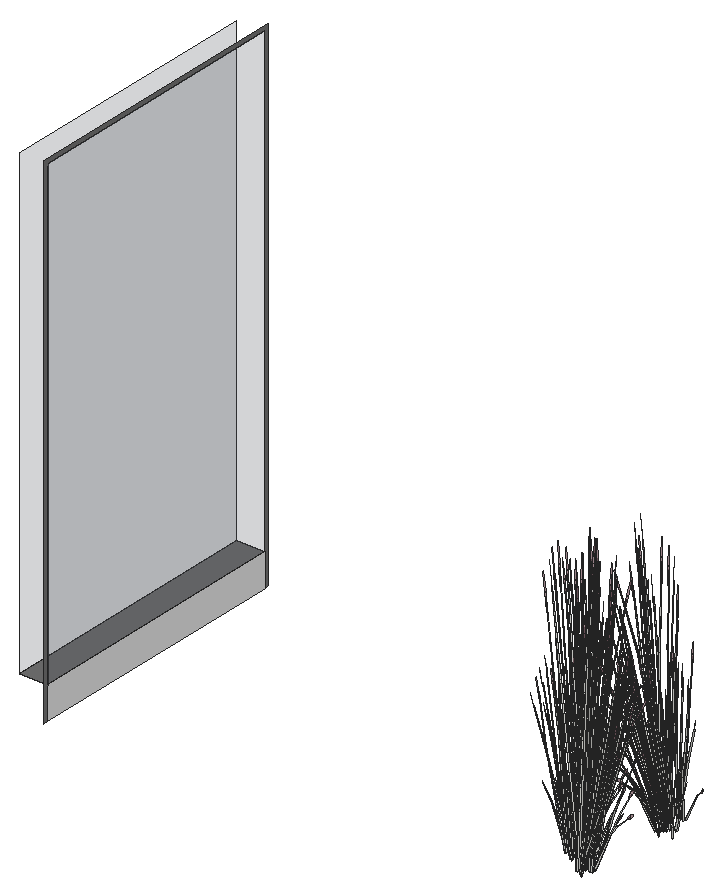
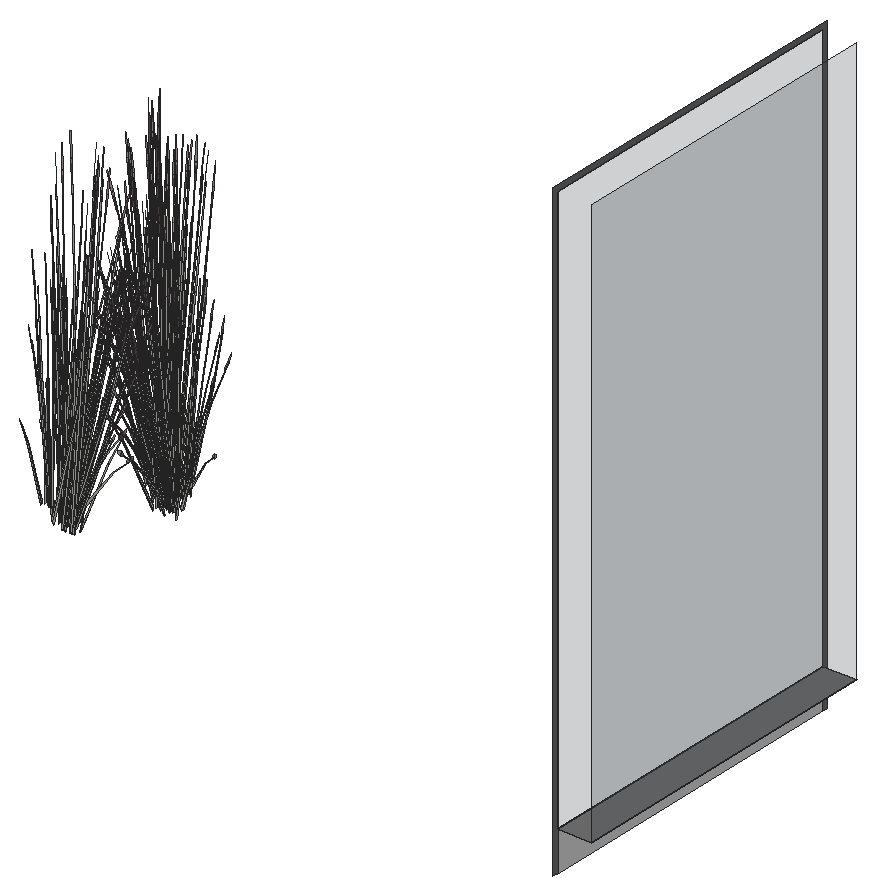
# SketchUp Ruby script. Lengths in inches.
U = 1.inch
M = Sketchup.active_model
def pt(a) = Geom::Point3d.new(a.map { |v| v * U })
def face(e, loops, mat)
  f = e.add_face(loops[0].map { |a| pt(a) })
  loops[1..].each { |l| e.add_face(l.map { |a| pt(a) }).erase! }
  f.material = f.back_material = mat if mat
  f
end
# faces: each face lists its corners as indices into pts; further lists are holes
def faces(e, pts, list, mat = nil) = list.each { |f| face(e, (f[0].is_a?(Array) ? f : [f]).map { |l| l.map { |i| pts[i] } }, mat) }
# xy, xz, yz: faces in a plane at the given z, y or x. An outline is a flat list of corners, or four numbers for a rectangle; further outlines are holes
def ring(l) = l.size == 4 ? [[l[0], l[1]], [l[2], l[1]], [l[2], l[3]], [l[0], l[3]]] : l.each_slice(2).to_a
def flat(e, list, mat, &to3) = list.each { |f| face(e, (f[0].is_a?(Array) ? f : [f]).map { |l| ring(l).map { |u, v| to3.(u, v) } }, mat) }
def xy(e, z, list, mat = nil) = flat(e, list, mat) { |x, y| [x, y, z] }
def xz(e, y, list, mat = nil) = flat(e, list, mat) { |x, z| [x, y, z] }
def yz(e, x, list, mat = nil) = flat(e, list, mat) { |y, z| [x, y, z] }
def lines(e, pts, list) = list.each { |a, b| e.add_line(pt(pts[a]), pt(pts[b])) }
# prism: a flat outline (further loops are holes) pulled along v
def prism(e, loops, v, mat = nil)
  f = face(e, loops, mat); d = Geom::Vector3d.new(v.map { |x| x * U })
  f.pushpull(f.normal.samedirection?(d) ? d.length : -d.length)
end
def box(e, o, s, mat = nil) = prism(e, [[o, [o[0] + s[0], o[1], o[2]], [o[0] + s[0], o[1] + s[1], o[2]], [o[0], o[1] + s[1], o[2]]]], [0, 0, s[2]], mat)
def at(x, y, z, deg = 0) = Geom::Transformation.translation(pt([x, y, z])) * Geom::Transformation.rotation(ORIGIN, Z_AXIS, deg.degrees)
def axes(o, x, y, z) = Geom::Transformation.new([*x, 0, *y, 0, *z, 0, *pt(o).to_a, 1])
def part(name) = M.definitions.add(name)
# library, detail: a bought-in or finely detailed component or shape, given as its bounding box
def library(name, o, s) = part(name).tap { |d| box(d.entities, o, s) }
def detail(e, o, s) = box(e.add_group.entities, o, s)
def put(e, d, t, mat = nil) = e.add_instance(d, t).tap { |i| i.material = mat if mat }
def group(e, t, mat = nil) = e.add_group.tap { |g| g.transformation = t; g.material = mat if mat }.entities
root = M.entities
M.materials.add("Glass_Basic_01").color = [105, 113, 122]
M.materials["Glass_Basic_01"].alpha = 0.25
M.materials.add("LightPink_Translucent").color = [144, 107, 117]
M.materials["LightPink_Translucent"].alpha = 0.75
M.materials.add("M01_Silver_Fog").color = [224, 224, 224]
M.materials.add("M06_Steel_Smoke").color = [114, 114, 114]
c1 = part("blade")
p = [[2.15,0.21,22],[0,0.17,0],[0.09,0.45,0],[2.18,0.31,22],[2.29,0.31,22],[0.38,0.45,0],
  [2.48,0.24,33],[2.49,0.24,33],[2.48,0.22,33]]
faces(c1.entities,p,[[0,1,2,3],[4,5,2,3],[6,3,4,7],[8,0,3,6]])
c2 = part("seeds")
p = [[0.3,-0.1,1.38],[-0.01,-0.03,1.59],[-0.01,-0.03,0.03],[0.14,-0.07,-0.07],[0.29,-0.03,3],[0.15,0.01,3.11]]
faces(c2.entities,p,[[0,1,2,3],[1,0,4,5]],"LightPink_Translucent")
c3 = part("blade with seeds")
put(c3.entities,c1,at(0,0,0))
put(c3.entities,c2,axes([2.4,0.25,30.99],[1.5799,-0.05474,1.17369],[-0.12525,1.92788,0.29478],[-0.07173,-0.02425,1.56792]))
xy(root,277,[[204,295,210,353]],"M06_Steel_Smoke")
yz(root,204,[[295,277,353,377]],"Glass_Basic_01")
yz(root,210,[[295,277,353,377]],"Glass_Basic_01")
yz(root,210,[[295,270,353,277]],"M01_Silver_Fog")
yz(root,210,[[294,270,295,270,295,377,353,377,353,270,354,270,354,378,294,378]],"M06_Steel_Smoke")
put(root,c3,axes([315.625,308.53,274.53],[0.41757,0.15024,-0.35414],[-0.12179,0.4383,0.4572],[0.16812,-0.04019,0.87481]))
put(root,c3,axes([311.76,309.83,272.02],[-0.47024,-0.26927,-0.49651],[0.28107,-0.48284,0],[-0.1071,-0.06133,1.57504]))
put(root,c3,axes([314.89,306.64,272.02],[0.47024,0.26927,-0.49651],[-0.28107,0.48284,0],[0.1071,0.06133,1.57504]))
put(root,c3,axes([310.72,307.83,274.53],[-0.41757,-0.15024,-0.35414],[0.12179,-0.4383,0.4572],[-0.16812,0.04019,0.87481]))
put(root,c3,axes([313.99,308.17,272.21],[0.56215,0,0],[0,0.55754,0],[0,0,1.78407]))
put(root,c3,axes([313.04,308.875,272.67],[-0.5073,0.35754,-0.29095],[-0.33735,-0.5052,-0.50002],[-0.12516,-0.05131,1.59708]))
put(root,c3,axes([314.15,306.87,272.47],[-0.53992,0.14294,0.17642],[-0.13332,-0.53195,0.35086],[0.04815,0.07751,1.60407]))
put(root,c3,axes([314.49,307.99,273.875],[-0.20841,0.0122,1.71376],[0.13825,-0.52864,0.13857],[0.297,0.0327,0.73262]))
put(root,c3,axes([314.75,306.84,272.03],[0.11803,0.46926,-0.30978],[-0.46876,0.13325,0.30978],[0.0945,0.05411,1.38974]))
put(root,c3,axes([315.5625,308.71,274.73],[0.18454,0.3672,0.0643],[-0.33652,0.17973,0.50621],[0.14834,-0.03546,0.77189]))
put(root,c3,axes([313.8125,307.89,272.38],[-0.63506,-0.11347,0.49198],[0.12924,-0.64083,0.19306],[0.09281,0.06188,1.70813]))
put(root,c3,axes([315.53,308.58,274.73],[-0.14195,0.49104,0.48003],[-0.46669,-0.16791,0.3958],[0.18353,-0.02951,0.9933]))
put(root,c3,axes([313.3,309.47,272.2],[-0.16394,-0.4643,0],[0.46814,-0.1626,0],[0,0,1.54371]))
put(root,c3,axes([312.99,309.03,272.62],[-0.09693,0.48062,0.1448],[-0.47357,-0.08343,-0.41347],[-0.08619,-0.04935,1.26744]))
put(root,c3,axes([311.16,307.78,275.05],[0.41757,0.15024,0.35414],[-0.12179,0.4383,-0.4572],[-0.16812,0.04019,0.87481]))
put(root,c3,axes([313.92,309.41,272.18],[0.5275,-0.18273,-0.19198],[0.18536,0.52636,0.00008],[0.05823,-0.0202,1.73897]))
put(root,c3,axes([314.1,309.625,272.47],[0.14515,-0.53522,0.17642],[0.53115,0.15146,0.35086],[-0.09175,0.00261,1.60407]))
put(root,c3,axes([313.98,308.41,272.21],[0.35073,0.34786,0],[-0.35073,0.34786,0],[0,0,1.69266]))
put(root,c3,axes([311.99,307.76,273.34],[0.14282,-0.0779,1.77064],[0.04925,0.54394,0.13857],[-0.30935,0.07218,0.63284]))
put(root,c3,axes([314.93,308.26,272.47],[-0.39477,-0.39228,0.17642],[0.39783,-0.38049,0.35086],[-0.0436,0.08011,1.60407]))
put(root,c3,axes([314.2,307.67,272.06],[0.52267,0.08829,-0.62353],[-0.11029,0.54463,-0.16365],[0.15598,0.06599,1.37633]))
put(root,c3,axes([316.51,308.62,272.77],[-0.31044,0.08891,1.1486],[0.14613,-0.36744,0.84392],[0.16469,0.02514,0.25299]))
put(root,c3,axes([313.1875,309.68,272.2],[-0.50654,-0.24178,0],[0.24378,-0.50239,0],[0,0,1.62707]))
put(root,c3,axes([313.61,309.04,272.46],[-0.49063,-0.43346,-0.25192],[0.41285,-0.48673,0.5513],[-0.13212,0.05071,1.68216]))
put(root,c3,axes([312.32,309.87,272.48],[0.47024,0.26927,0.49651],[-0.28107,0.48284,0],[-0.1071,-0.06133,1.57504]))
put(root,c3,axes([313.98,308.01,272.72],[0.24378,-0.48527,0.44739],[0.50654,0.23354,-0.21531],[0,0.11186,1.43643]))
put(root,c3,axes([316.36,310.17,274.71],[-0.04543,-0.04715,1.77383],[0.09938,-0.50538,-0.16761],[0.17896,-0.03229,0.31391]))
put(root,c3,axes([310.45,308.125,274.72],[-0.08205,0.06992,1.74944],[0.00698,0.51086,-0.27667],[-0.18807,0.06644,0.14031]))
put(root,c3,axes([313.88,308.28,272.29],[0,0.62282,-0.05637],[-0.62828,0,0],[0,0.01957,1.79368]))
put(root,c3,axes([311,308.06,274.68],[-0.13612,0.48987,-0.51099],[-0.46669,-0.16791,-0.3958],[-0.1879,0.04492,0.97773]))
put(root,c3,axes([310.98,307.64,275.03],[0.25281,0.48765,-0.1216],[-0.44869,0.23964,-0.67495],[-0.18908,0.06434,1.02557]))
put(root,c3,axes([313.93,307.84,272.21],[0.30184,0.45202,-0.44739],[-0.45719,0.31831,0.21531],[0.09768,0.05593,1.43643]))
put(root,c3,axes([315.97,309.75,273.93],[-0.09617,-0.45271,-0.03492],[0.45453,-0.10408,-0.15832],[0.09492,0.0287,0.52218]))
put(root,c3,axes([312.05,310.15,272.375],[-0.31414,0.53965,0],[-0.52557,-0.30095,-0.51607],[-0.1197,-0.06854,1.63711]))
put(root,c3,axes([314.79,309.74,275.03],[0.0269,-0.54769,-0.1216],[0.50939,0.01497,-0.67495],[0.19618,0.03804,1.02557]))
put(root,c3,axes([315.26,308.28,272.48],[0,-0.53854,0.49651],[0.56215,0,0],[0,0.12266,1.57504]))
put(root,c3,axes([313.85,308.68,272.72],[0.54562,-0.03324,0.44739],[0.04934,0.55185,-0.21531],[-0.09768,0.05593,1.43643]))
put(root,c3,axes([314.1875,308.12,272.62],[0.46814,-0.15705,0.1448],[0.16394,0.44848,-0.41347],[0,0.0987,1.26744]))
put(root,c3,axes([314.71,309.52,275.05],[-0.28589,-0.33718,0.35414],[0.32644,-0.31919,-0.4572],[0.16586,0.04856,0.87481]))
put(root,c3,axes([313.36,308.95,272.21],[-0.54562,0.03324,-0.44739],[-0.04934,-0.55185,0.21531],[-0.09768,0.05593,1.43643]))
put(root,c3,axes([315.93,309.21,272.59],[-0.12101,-0.13245,1.43002],[0.15744,-0.43816,-0.30754],[0.24483,0.05936,0.61141]))
put(root,c3,axes([313.76,309.69,272.2],[0.50654,0.24178,0],[-0.24378,0.50239,0],[0,0,1.74954]))
put(root,c3,axes([315.23,309.41,274.72],[0.10779,-0.00911,1.74944],[0.29564,-0.41839,-0.27667],[0.19172,0.05523,0.14031]))
put(root,c3,axes([313.97,310.23,272.19],[-0.31023,-0.54153,-0.05142],[0.52557,-0.30095,0.51607],[-0.12951,0.05156,1.6363]))
put(root,c3,axes([313.86,308.92,272.62],[0.37121,0.32357,0.1448],[-0.30963,0.36505,-0.41347],[-0.08619,0.04935,1.26744]))
put(root,c3,axes([310.92,309,274.73],[-0.12461,-0.49565,0.48003],[0.48882,-0.08602,0.3958],[-0.14406,0.11657,0.9933]))
put(root,c3,axes([310.83,308.91,274.73],[-0.34493,-0.22649,0.0643],[0.20082,-0.32253,0.50621],[-0.11059,0.10427,0.77189]))
put(root,c3,axes([310.99,308.31,273.875],[0.17434,-0.11391,1.71376],[0.14677,0.52637,0.13857],[-0.27369,0.11897,0.73262]))
put(root,c3,axes([314.82,309.48,274.98],[0.50227,0.01297,-0.71045],[-0.03373,0.54602,0.08574],[0.21278,0.05762,1.00501]))
put(root,c3,axes([314.25,309.91,272.48],[0.47024,-0.26927,0.49651],[0.28107,0.48284,0],[-0.1071,0.06133,1.57504]))
put(root,c3,axes([313.58,309.49,272.29],[0.21845,0.61869,-0.06012],[-0.62418,0.21679,0],[0.00763,0.02161,1.72173]))
put(root,c3,axes([313.82,310.16,272.03],[-0.46876,-0.13325,-0.30978],[0.11803,-0.46926,0.30978],[-0.0945,0.05411,1.38974]))
put(root,c3,axes([310.44,309.21,272.59],[0.17462,0.04421,1.43002],[0.11254,0.45156,-0.30754],[-0.23719,0.08453,0.61141]))
put(root,c3,axes([311.22,308.84,275.05],[0.43736,-0.07697,0.35414],[0.11549,0.43998,-0.4572],[-0.12533,0.11818,0.87481]))
put(root,c3,axes([315.64,308.37,272.375],[0.62828,0,0],[0,0.6019,-0.51607],[0,0.13709,1.63711]))
put(root,c3,axes([309.54,308.64,274.71],[0.06412,0.01444,1.77383],[0.19837,0.47583,-0.16761],[-0.13126,0.12489,0.31391]))
put(root,c3,axes([315.39,308.68,272.2],[-0.62797,-0.00431,-0.04976],[0,-0.6019,0.49943],[-0.01973,0.13702,1.58352]))
put(root,c3,axes([314.03,308.15,272.67],[0.56585,0.25696,-0.29095],[-0.27246,0.54236,-0.50002],[0.01778,0.13316,1.59708]))
put(root,c3,axes([310.08,310.15,272.77],[0.2094,-0.24408,1.1486],[0.08263,0.38639,0.84392],[-0.15132,0.06919,0.25299]))
put(root,c3,axes([315.12,309.7,274.53],[0.28589,0.33718,-0.35414],[-0.32644,0.31919,0.4572],[0.16586,0.04856,0.87481]))
put(root,c3,axes([315.26,308.76,272.03],[-0.35073,0.33601,-0.30978],[-0.35073,-0.33601,0.30978],[0,0.10823,1.38974]))
put(root,c3,axes([313.74,308.8,272.67],[0.05855,0.61451,-0.29095],[-0.60981,0.03716,-0.50002],[-0.10738,0.08185,1.59708]))
put(root,c3,axes([314.97,309.83,274.73],[-0.0253,0.40952,0.0643],[-0.38204,-0.01123,0.50621],[0.14634,0.04285,0.77189]))
put(root,c3,axes([313.97,308.56,272.21],[-0.24378,0.48527,-0.44739],[-0.50654,-0.23354,0.21531],[0,0.11186,1.43643]))
put(root,c3,axes([310.87,309.1,274.53],[-0.43736,0.07697,-0.35414],[-0.11549,-0.43998,0.4572],[-0.12533,0.11818,0.87481]))
put(root,c3,axes([315.01,309.7,274.73],[-0.37048,0.35486,0.48003],[-0.31952,-0.37685,0.3958],[0.17382,0.06546,0.9933]))
put(root,c3,axes([310.23,310.09,275.65],[0.44338,0.14375,-0.06488],[-0.13639,0.44245,-0.29416],[-0.07252,0.06718,0.97024]))
put(root,c3,axes([313.38,309.27,272.06],[-0.33843,0.40479,-0.62353],[-0.42041,-0.36705,-0.16365],[-0.13561,0.10098,1.37633]))
put(root,c3,axes([313.83,310.11,275.05],[-0.0776,-0.43378,0.35414],[0.44361,-0.11454,-0.4572],[0.11915,0.12431,0.87481]))
put(root,c3,axes([313.98,309.95,272.33],[0.62903,0.17504,0.30756],[-0.15737,0.62568,-0.36492],[-0.10411,0.07831,1.64885]))
put(root,c3,axes([313.93,310.37,272.02],[-0.47024,0.26927,-0.49651],[-0.28107,-0.48284,0],[-0.1071,0.06133,1.57504]))
put(root,c3,axes([315.5,308.78,272.02],[0,0.53854,-0.49651],[-0.56215,0,0],[0,0.12266,1.57504]))
put(root,c3,axes([314.09,308.84,273.875],[-0.18664,-0.09279,1.71376],[0.38624,-0.38925,0.13857],[0.24072,0.1756,0.73262]))
put(root,c3,axes([314.13,307.61,274.47],[-0.43417,-0.27982,1.38283],[0.45844,-0.43566,0.59665],[0.14008,0.26255,1.33663]))
put(root,c3,axes([311,308.8,275.03],[0.46478,0.29695,-0.1216],[-0.26776,0.43004,-0.67495],[-0.13131,0.14949,1.02557]))
put(root,c3,axes([314.78,309.89,272.77],[-0.2829,-0.15485,1.1486],[0.36529,-0.15734,0.84392],[0.09853,0.13328,0.25299]))
put(root,c3,axes([313.79,310.33,275.03],[0.2994,-0.46097,-0.1216],[0.43359,0.26557,-0.67495],[0.15072,0.13024,1.02557]))
put(root,c3,axes([311.625,308.66,273.875],[0.1255,-0.16547,1.71376],[0.31687,0.44665,0.13857],[-0.21734,0.2034,0.73262]))
put(root,c3,axes([311.23,309.15,274.68],[0.12908,0.49174,-0.51099],[-0.48882,0.08602,-0.3958],[-0.14008,0.13208,0.97773]))
put(root,c3,axes([311.82,309.71,275.05],[0.33997,-0.28354,0.35414],[0.32182,0.32376,-0.4572],[-0.04897,0.1645,0.87481]))
put(root,c3,axes([314.36,310.29,272.375],[0.31414,0.53965,0],[-0.52557,0.30095,-0.51607],[-0.1197,0.06854,1.63711]))
put(root,c3,axes([313.4,310.72,274.71],[0.00149,-0.0652,1.77383],[0.43058,-0.28766,-0.16761],[0.14956,0.10267,0.31391]))
put(root,c3,axes([314.86,310.47,271.49],[0.03661,-0.07775,1.76342],[0.46087,-0.22898,-0.26939],[0.13972,0.11851,0.30037]))
put(root,c3,axes([314.09,308.15,272.84],[-0.01373,-0.50706,1.41272],[0.62119,0.13144,0.59816],[-0.14692,0.27746,1.3335]))
put(root,c3,axes([314.25,308.7,272.09],[0.18424,0.49308,-0.69212],[-0.53071,0.17758,-0.18165],[0.02036,0.16697,1.52773]))
put(root,c3,axes([311.51,309.97,274.73],[-0.4129,-0.02509,0.0643],[0.01132,-0.37891,0.50621],[-0.04321,0.14514,0.77189]))
put(root,c3,axes([310.63,310.4,271.49],[0.0674,0.0538,1.76342],[0.11428,0.49852,-0.26939],[-0.14937,0.10631,0.30037]))
put(root,c3,axes([311.64,310,274.73],[-0.35779,-0.36745,0.48003],[0.37996,-0.3169,0.3958],[-0.066,0.17239,0.9933]))
put(root,c3,axes([314.14,310.11,274.68],[0.4958,-0.12802,-0.51099],[0.08673,0.48481,-0.3958],[0.13317,0.13893,0.97773]))
put(root,c3,axes([312.77,310.18,275.05],[0.15148,-0.41415,0.35414],[0.44193,0.12079,-0.4572],[0.04052,0.16674,0.87481]))
put(root,c3,axes([314.83,310.6,272.67],[-0.3222,-0.01689,1.0506],[0.21278,-0.35872,0.58006],[0.12729,0.12745,0.8241]))
put(root,c3,axes([313.9,310.5,274.73],[-0.22836,0.34211,0.0643],[-0.3252,-0.19918,0.50621],[0.10513,0.10968,0.77189]))
put(root,c3,axes([313.36,311.66,275.65],[0.34721,-0.30895,-0.06488],[0.31814,0.33837,-0.29416],[0.0224,0.09588,0.97024]))
put(root,c3,axes([314,310.41,274.73],[-0.49974,0.12359,0.48003],[-0.08673,-0.48481,0.3958],[0.11753,0.14288,0.9933]))
put(root,c3,axes([311.53,309.07,273.875],[0.09355,-0.18511,1.71376],[0.39247,0.38307,0.13857],[-0.17705,0.23875,0.73262]))
put(root,c3,axes([313.78,309.73,272.59],[0.00887,-0.17852,1.43002],[0.42372,-0.19941,-0.30754],[0.1308,0.21367,0.61141]))
put(root,c3,axes([312.63,310.55,274.73],[-0.37023,0.18303,0.0643],[-0.18122,-0.33376,0.50621],[0.03575,0.14712,0.77189]))
put(root,c3,axes([311.64,310.11,274.53],[-0.33997,0.28354,-0.35414],[-0.32182,-0.32376,0.4572],[-0.04897,0.1645,0.87481]))
put(root,c3,axes([310.47,310.03,274.72],[-0.01249,0.10657,1.74944],[0.35444,0.37075,-0.27667],[-0.09279,0.17532,0.14031]))
put(root,c3,axes([311.6,309.79,275.4],[0.55221,0.02668,-0.13498],[-0.01509,0.50521,-0.74919],[-0.03836,0.19458,1.13838]))
put(root,c3,axes([312.62,310.35,275.03],[0.49168,-0.25073,-0.1216],[0.24162,0.44501,-0.67495],[0.06487,0.18753,1.02557]))
put(root,c3,axes([312.76,310.52,275.0625],[-0.4951,-0.14079,0.53283],[0.1693,-0.46287,0.43934],[0.02975,0.18203,1.10256]))
put(root,c3,axes([311.85,311.22,272.77],[-0.013,-0.32022,1.1486],[0.32493,0.22839,0.84392],[-0.0639,0.15263,0.25299]))
put(root,c3,axes([312.71,310.45,271.49],[0.08132,-0.0293,1.76342],[0.48914,0.1613,-0.26939],[0.0143,0.18179,0.30037]))
put(root,c3,axes([311.98,309.98,275],[0.35968,0.36185,-0.5672],[-0.37996,0.3169,-0.43934],[-0.05473,0.18385,1.08528]))
put(root,c3,axes([311.59,310.52,272.82],[0.45645,-0.09537,0.06507],[0.10494,0.38421,-0.86304],[-0.02894,0.19449,0.7736]))
put(root,c3,axes([313.04,310.33,274.68],[0.49392,0.135,-0.51099],[-0.1693,0.46287,-0.3958],[0.04529,0.18636,0.97773]))
put(root,c3,axes([313.32,309.375,273.875],[-0.11485,-0.17291,1.71376],[0.53072,-0.14557,0.13857],[0.11995,0.27145,0.73262]))
put(root,c3,axes([312.82,310.62,274.53],[-0.15148,0.41415,-0.35414],[-0.44193,-0.12079,0.4572],[0.04052,0.16674,0.87481]))
put(root,c3,axes([311.86,309.81,275.34],[-0.01307,0.49815,-0.7886],[-0.55054,-0.03346,0.09517],[-0.0581,0.21104,1.11556]))
put(root,c3,axes([310.43,311.125,274.71],[0.057,-0.03251,1.77383],[0.47114,0.21627,-0.16761],[-0.01107,0.18007,0.31391]))
put(root,c3,axes([312.38,309.46,273.875],[-0.0123,-0.2067,1.71376],[0.53301,0.13712,0.13857],[-0.03297,0.29456,0.73262]))
put(root,c3,axes([312.86,310.24,274.98],[0.23981,0.43789,-0.71045],[-0.49365,0.24404,0.08574],[0.05608,0.21158,1.00501]))
put(root,c3,axes([311.47,310.93,272.59],[0.15856,-0.08496,1.43002],[0.39147,0.25616,-0.30754],[-0.11652,0.22165,0.61141]))
put(root,c3,axes([312.5,311.35,274.72],[0.06369,0.08672,1.74944],[0.51399,0.03407,-0.27667],[0.05169,0.19126,0.14031]))
put(root,c3,axes([311.68,310.52,273.36],[0.01104,-0.27801,1.54345],[0.49652,0.14685,0.21329],[-0.04302,0.2963,0.72882]))
put(root,c3,axes([317.4,324.24,275.875],[0.11485,0.17291,1.71376],[-0.53072,0.14557,0.13857],[-0.11995,-0.27145,0.73262]))
put(root,c3,axes([318.28,323.09,276.72],[-0.07685,-0.07551,1.74944],[-0.51287,0.04787,-0.27667],[-0.08185,-0.1806,0.14031]))
put(root,c3,axes([319.47,323.99,274.59],[-0.14282,0.10901,1.43002],[-0.42773,-0.19079,-0.30754],[0.07929,-0.23728,0.61141]))
put(root,c3,axes([318.82,324.37,276.98],[-0.23981,-0.43789,-0.71045],[0.49365,-0.24404,0.08574],[-0.05608,-0.21158,1.00501]))
put(root,c3,axes([317.26,323.78,274.59],[-0.03043,0.17617,1.43002],[-0.4448,0.14748,-0.30754],[-0.10397,-0.22771,0.61141]))
put(root,c3,axes([318.4,323.4,273.49],[-0.08428,0.0194,1.76342],[-0.46606,-0.21841,-0.26939],[0.00782,-0.18218,0.30037]))
put(root,c3,axes([319.82,324.8,276.98],[0.01307,-0.49815,-0.71045],[0.55054,0.03346,0.08574],[0.0581,-0.21104,1.00501]))
put(root,c3,axes([320.58,324.02,276.72],[-0.00485,-0.10718,1.74944],[-0.40965,-0.30977,-0.27667],[0.06333,-0.18778,0.14031]))
put(root,c3,axes([318.86,324,276.53],[0.15148,-0.41415,-0.35414],[0.44193,0.12079,0.4572],[-0.04052,-0.16674,0.87481]))
put(root,c3,axes([319.2,324.55,275.875],[-0.09355,0.18511,1.71376],[-0.39247,-0.38307,0.13857],[0.17705,-0.23875,0.73262]))
put(root,c3,axes([320.47,323.64,276.71],[-0.05103,0.04113,1.77383],[-0.49994,-0.13878,-0.16761],[-0.0181,-0.17951,0.31391]))
put(root,c3,axes([318.64,324.28,276.68],[-0.49392,-0.135,-0.51099],[0.1693,-0.46287,-0.3958],[-0.04529,-0.18636,0.97773]))
put(root,c3,axes([318.94,323.12,274.77],[0.06446,0.31404,1.1486],[-0.35756,-0.17393,0.84392],[0.03848,-0.1608,0.25299]))
put(root,c3,axes([319.7,324.63,276.68],[-0.35968,-0.36185,-0.51099],[0.37996,-0.3169,-0.3958],[0.05473,-0.18385,0.97773]))
put(root,c3,axes([317.75,322.85,276.71],[-0.00937,0.06455,1.77383],[-0.46231,0.23427,-0.16761],[-0.13604,-0.11975,0.31391]))
put(root,c3,axes([317.65,323.99,277.09],[0.55971,-0.13842,0.53763],[0.09714,0.54299,0.4433],[-0.13164,-0.16003,1.11249]))
put(root,c3,axes([318.92,324.09,276.73],[0.4951,0.14079,0.48003],[-0.1693,0.46287,0.3958],[-0.02975,-0.18203,0.9933]))
put(root,c3,axes([319.06,324.26,277.03],[-0.49168,0.25073,-0.1216],[-0.24162,-0.44501,-0.67495],[-0.06487,-0.18753,1.02557]))
put(root,c3,axes([320.08,324.82,277.03],[-0.55221,-0.02668,-0.1216],[0.01509,-0.50521,-0.67495],[0.03836,-0.19458,1.02557]))
put(root,c3,axes([320.04,324.5,276.53],[0.33997,-0.28354,-0.35414],[0.32182,0.32376,0.4572],[0.04897,-0.1645,0.87481]))
put(root,c3,axes([317.1,323.5,274.77],[0.2621,0.18744,1.1486],[-0.38171,0.11267,0.84392],[-0.08167,-0.14405,0.25299]))
put(root,c3,axes([319.05,324.06,276.73],[0.37023,-0.18303,0.0643],[0.18122,0.33376,0.50621],[-0.03575,-0.14712,0.77189]))
put(root,c3,axes([317.74,324.49,276.98],[-0.42844,-0.2603,-0.71045],[0.30448,-0.45614,0.08574],[-0.15523,-0.15542,1.00501]))
put(root,c3,axes([317.59,324.15,276.53],[-0.0776,-0.43378,-0.35414],[0.44361,-0.11454,0.4572],[-0.11915,-0.12431,0.87481]))
put(root,c3,axes([317.78,324.11,276.73],[0.22836,-0.34211,0.0643],[0.3252,0.19918,0.50621],[-0.10513,-0.10968,0.77189]))
put(root,c3,axes([316.9,324.07,273.49],[-0.04867,0.07094,1.76342],[-0.49185,0.15296,-0.26939],[-0.11882,-0.13915,0.30037]))
put(root,c3,axes([317.71,326.01,274.1],[-0.20635,-0.55225,-0.69835],[0.59439,-0.19889,-0.18329],[-0.02281,-0.18701,1.54149]))
put(root,c3,axes([316.63,324.78,275.875],[0.18664,0.09279,1.71376],[-0.38624,0.38925,0.13857],[-0.24072,-0.1756,0.73262]))
put(root,c3,axes([320.47,324.33,273.49],[-0.0752,-0.04243,1.76342],[-0.19317,-0.47398,-0.26939],[0.13031,-0.12863,0.30037]))
put(root,c3,axes([318.91,324.43,277.05],[-0.15148,0.41415,0.35414],[-0.44193,-0.12079,-0.4572],[-0.04052,-0.16674,0.87481]))
put(root,c3,axes([317.54,324.51,276.68],[-0.4958,0.12802,-0.51099],[-0.08673,-0.48481,-0.3958],[-0.13317,-0.13893,0.97773]))
put(root,c3,axes([320.04,324.61,276.73],[0.35779,0.36745,0.48003],[-0.37996,0.3169,0.3958],[0.066,-0.17239,0.9933]))
put(root,c3,axes([317.88,324.07,277.43],[-0.33533,0.51628,-0.13619],[-0.48563,-0.29744,-0.75594],[-0.16881,-0.14586,1.14864]))
put(root,c3,axes([320.17,324.64,276.73],[0.4129,0.02509,0.0643],[-0.01132,0.37891,0.50621],[0.04321,-0.14514,0.77189]))
put(root,c3,axes([319.86,324.9,277.05],[-0.33997,0.28354,0.35414],[-0.32182,-0.32376,-0.4572],[0.04897,-0.1645,0.87481]))
put(root,c3,axes([320.46,325.66,276.98],[0.26246,-0.42493,-0.71045],[0.45991,0.30199,0.08574],[0.15671,-0.15395,1.00501]))
put(root,c3,axes([317.63,324.43,274.375],[-0.31414,-0.53965,0],[0.52557,-0.30095,-0.51607],[0.1197,-0.06854,1.63711]))
put(root,c3,axes([320.45,325.47,276.68],[-0.12908,-0.49174,-0.51099],[0.48882,-0.08602,-0.3958],[0.14008,-0.13208,0.97773]))
put(root,c3,axes([318.32,323.78,274.13],[-0.34721,0.30895,-0.03893],[-0.31814,-0.33837,-0.17649],[-0.0224,-0.09588,0.58215]))
put(root,c3,axes([316.6,323.93,276.72],[-0.10811,-0.0038,1.74944],[-0.34418,0.38014,-0.27667],[-0.18364,-0.07767,0.14031]))
put(root,c3,axes([320.68,325.82,277.03],[-0.46478,-0.29695,-0.1216],[0.26776,-0.43004,-0.67495],[0.13131,-0.14949,1.02557]))
put(root,c3,axes([318.76,327.4375,275.33],[0.4342,0.21716,1.51261],[-0.42537,0.46784,0.59816],[-0.19053,-0.27728,1.26806]))
put(root,c3,axes([317.85,324.5,277.05],[0.0776,0.43378,0.35414],[-0.44361,0.11454,-0.4572],[-0.11915,-0.12431,0.87481]))
put(root,c3,axes([316.49,325.9375,274.02],[0,-0.53854,-0.49651],[0.56215,0,0],[0,-0.12266,1.57504]))
put(root,c3,axes([318.05,324.34,274.02],[0.47024,-0.26927,-0.49651],[0.28107,0.48284,0],[0.1071,-0.06133,1.57504]))
put(root,c3,axes([320.84,325.27,274.59],[-0.1795,-0.01595,1.43002],[-0.18389,-0.42791,-0.30754],[0.22051,-0.12105,0.61141]))
put(root,c3,axes([316.52,324.79,277.09],[0.41494,-0.39744,0.53763],[0.35786,0.42207,0.4433],[-0.19468,-0.07331,1.11249]))
put(root,c3,axes([321.83,325.6875,276.71],[-0.06563,-0.00409,1.77383],[-0.27252,-0.43825,-0.16761],[0.10944,-0.1441,0.31391]))
put(root,c3,axes([318.61,325.45,274.06],[0.33843,-0.40479,-0.62353],[0.42041,0.36705,-0.16365],[0.13561,-0.10098,1.37633]))
put(root,c3,axes([321.05,324.49,274.77],[-0.16736,0.27414,1.1486],[-0.14385,-0.36832,0.84392],[0.13822,-0.09229,0.25299]))
put(root,c3,axes([320.8125,325.52,276.53],[0.43736,-0.07697,-0.35414],[0.11549,0.43998,0.4572],[0.12533,-0.11818,0.87481]))
put(root,c3,axes([316.71,324.78,276.73],[0.0253,-0.40952,0.0643],[0.38204,0.01123,0.50621],[-0.14634,-0.04285,0.77189]))
put(root,c3,axes([318.02,326.16,274.21],[0.24378,-0.48527,-0.44739],[0.50654,0.23354,0.21531],[0,-0.11186,1.43643]))
put(root,c3,axes([316.5625,324.91,276.53],[-0.28589,-0.33718,-0.35414],[0.32644,-0.31919,0.4572],[-0.16586,-0.04856,0.87481]))
put(root,c3,axes([318.24,325.92,274.67],[-0.05855,-0.61451,-0.29095],[0.60981,-0.03716,-0.50002],[0.10738,-0.08185,1.59708]))
put(root,c3,axes([316.73,325.95,274.03],[0.35073,-0.33601,-0.30978],[0.35073,0.33601,0.30978],[0,-0.10823,1.38974]))
put(root,c3,axes([316.59,324.34,274.13],[-0.14494,0.43975,-0.03893],[-0.4461,-0.13527,-0.17649],[-0.06773,-0.07192,0.58215]))
put(root,c3,axes([320.46,325.78,277.05],[-0.43736,0.07697,0.35414],[-0.11549,-0.43998,-0.4572],[0.12533,-0.11818,0.87481]))
put(root,c3,axes([317.96,326.5625,274.67],[-0.56585,-0.25696,-0.29095],[0.27246,-0.54236,-0.50002],[-0.01778,-0.13316,1.59708]))
put(root,c3,axes([316.35,326.35,274.375],[-0.62828,0,0],[0,-0.6019,-0.51607],[0,-0.13709,1.63711]))
put(root,c3,axes([316.46,325.27,274.59],[0.0981,0.14994,1.43002],[-0.22605,0.40756,-0.30754],[-0.23211,-0.09741,0.61141]))
put(root,c3,axes([318.16,324.56,274.03],[0.46876,0.13325,-0.30978],[-0.11803,0.46926,0.30978],[0.0945,-0.05411,1.38974]))
put(root,c3,axes([316.86,325.14,276.98],[-0.50227,-0.01297,-0.71045],[0.03373,-0.54602,0.08574],[-0.21278,-0.05762,1.00501]))
put(root,c3,axes([320.85,325.71,276.73],[0.34493,0.22649,0.0643],[-0.20082,0.32253,0.50621],[0.11059,-0.10427,0.77189]))
put(root,c3,axes([320.76,325.61,276.73],[0.12461,0.49565,0.48003],[-0.48882,0.08602,0.3958],[0.14406,-0.11657,0.9933]))
put(root,c3,axes([322.07,326.21,276.72],[0.06972,-0.08203,1.74944],[-0.08924,-0.50318,-0.27667],[0.17494,-0.0954,0.14031]))
put(root,c3,axes([316.84,326.1875,274.33],[-0.46736,0.45277,0.30756],[-0.46764,-0.44801,-0.36492],[-0.01632,-0.12858,1.64885]))
